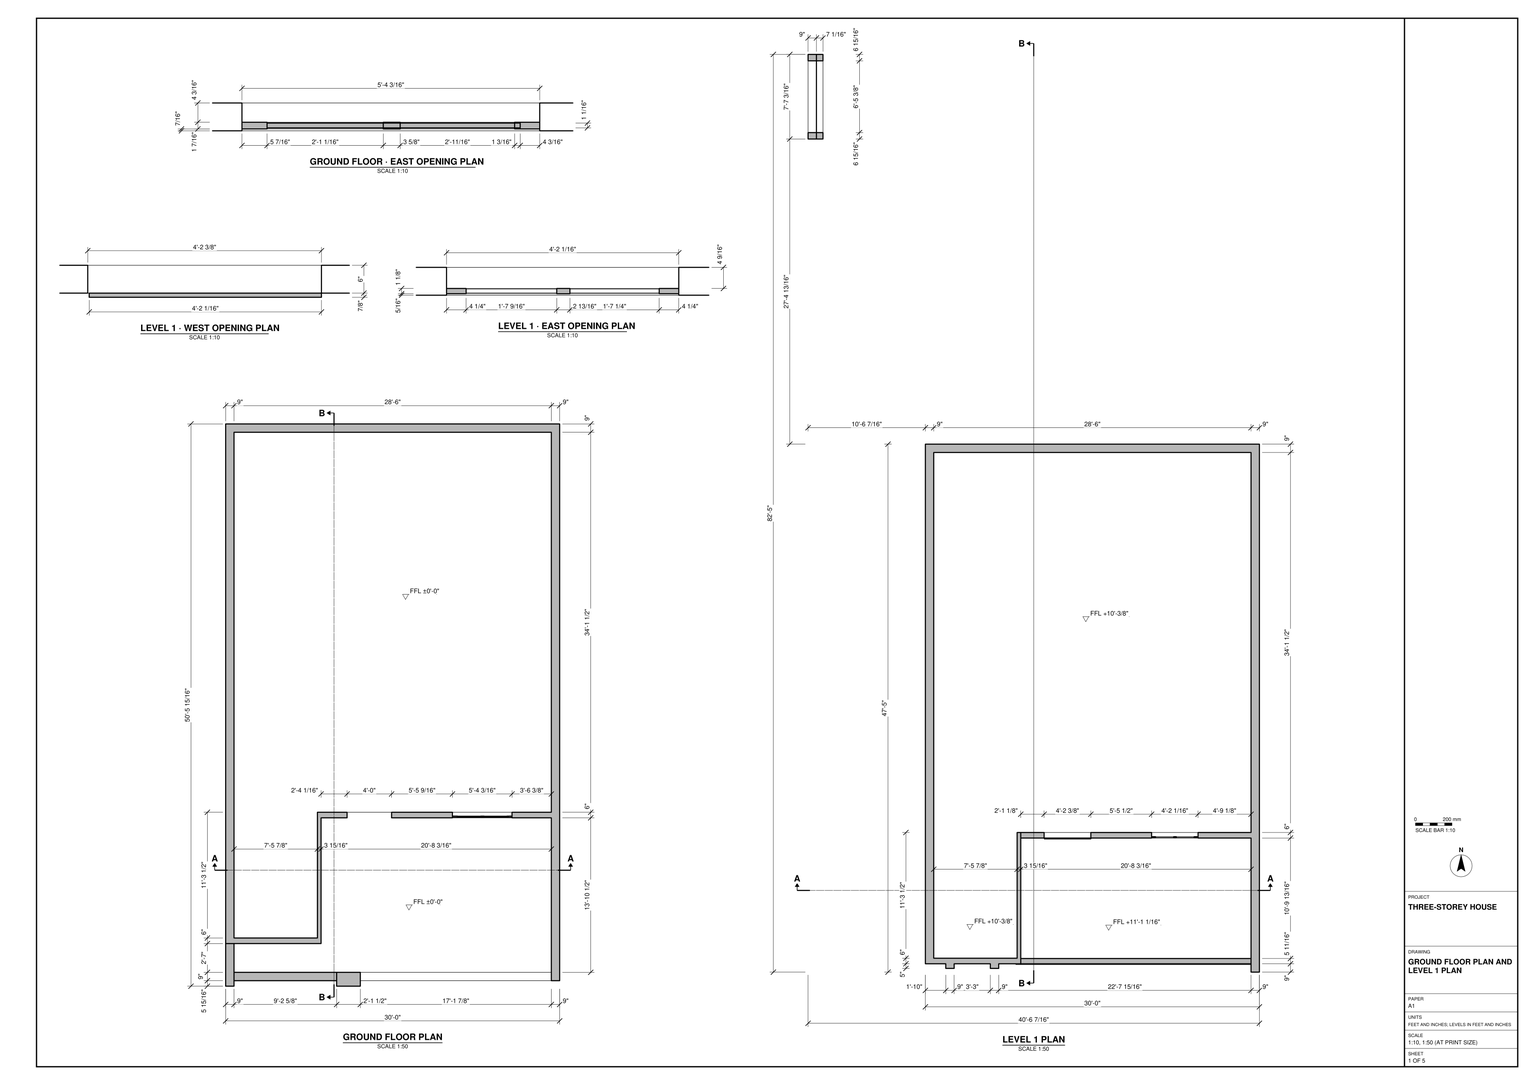
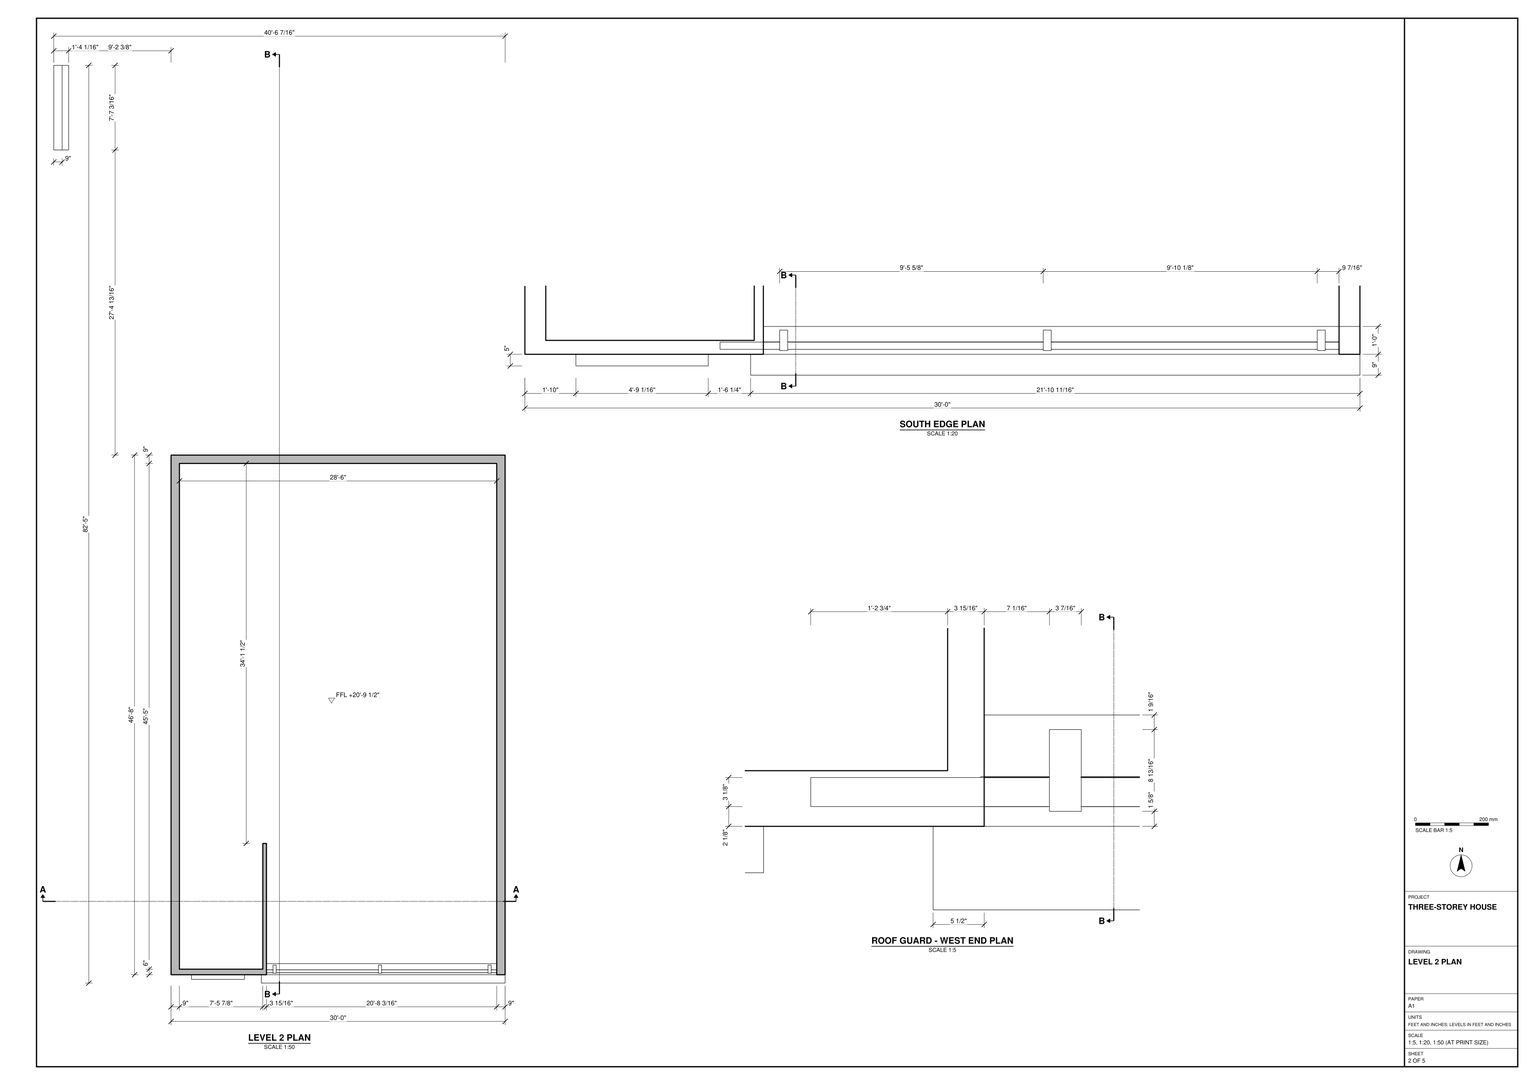
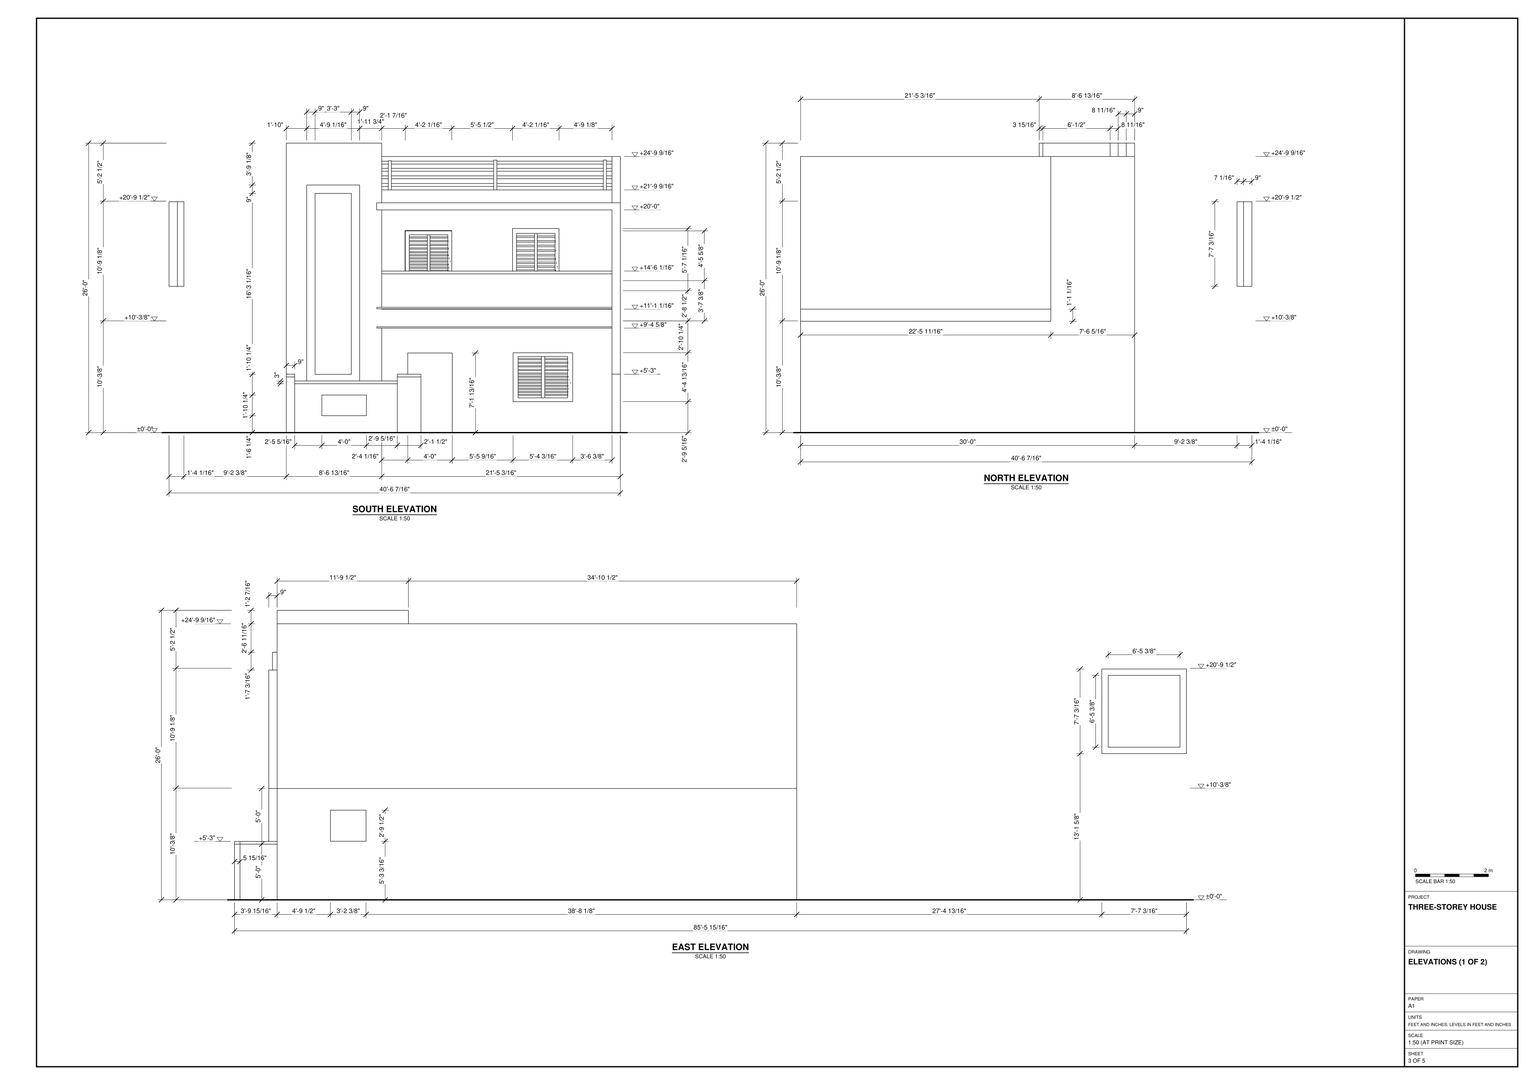
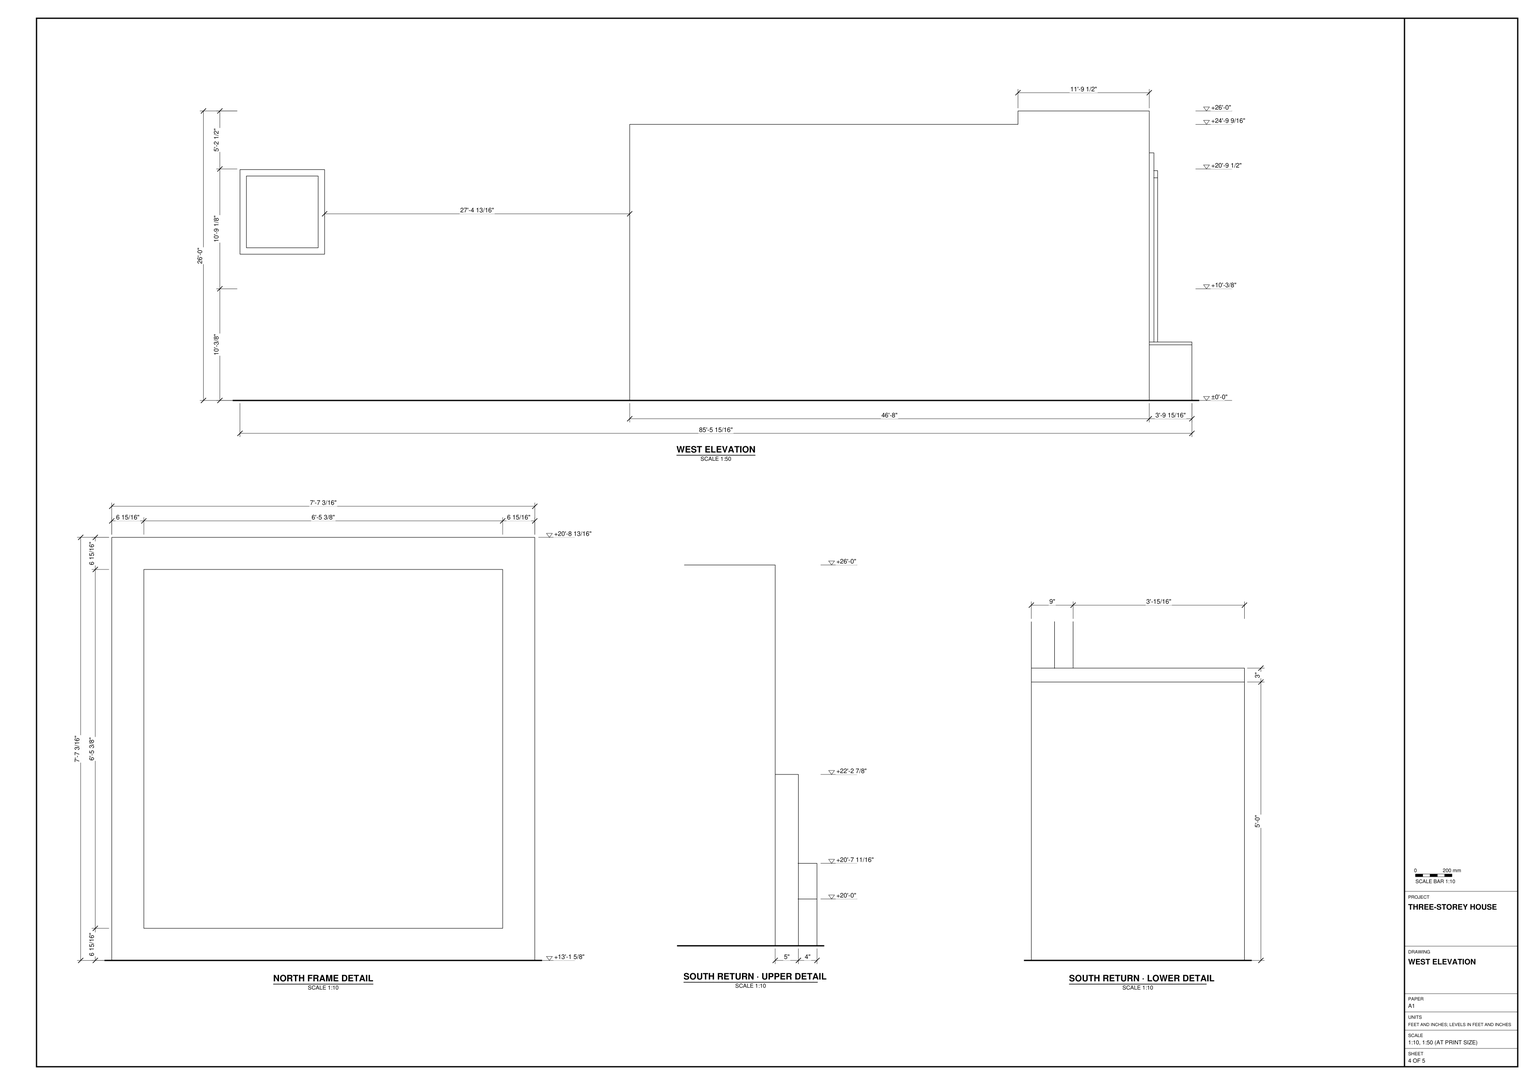
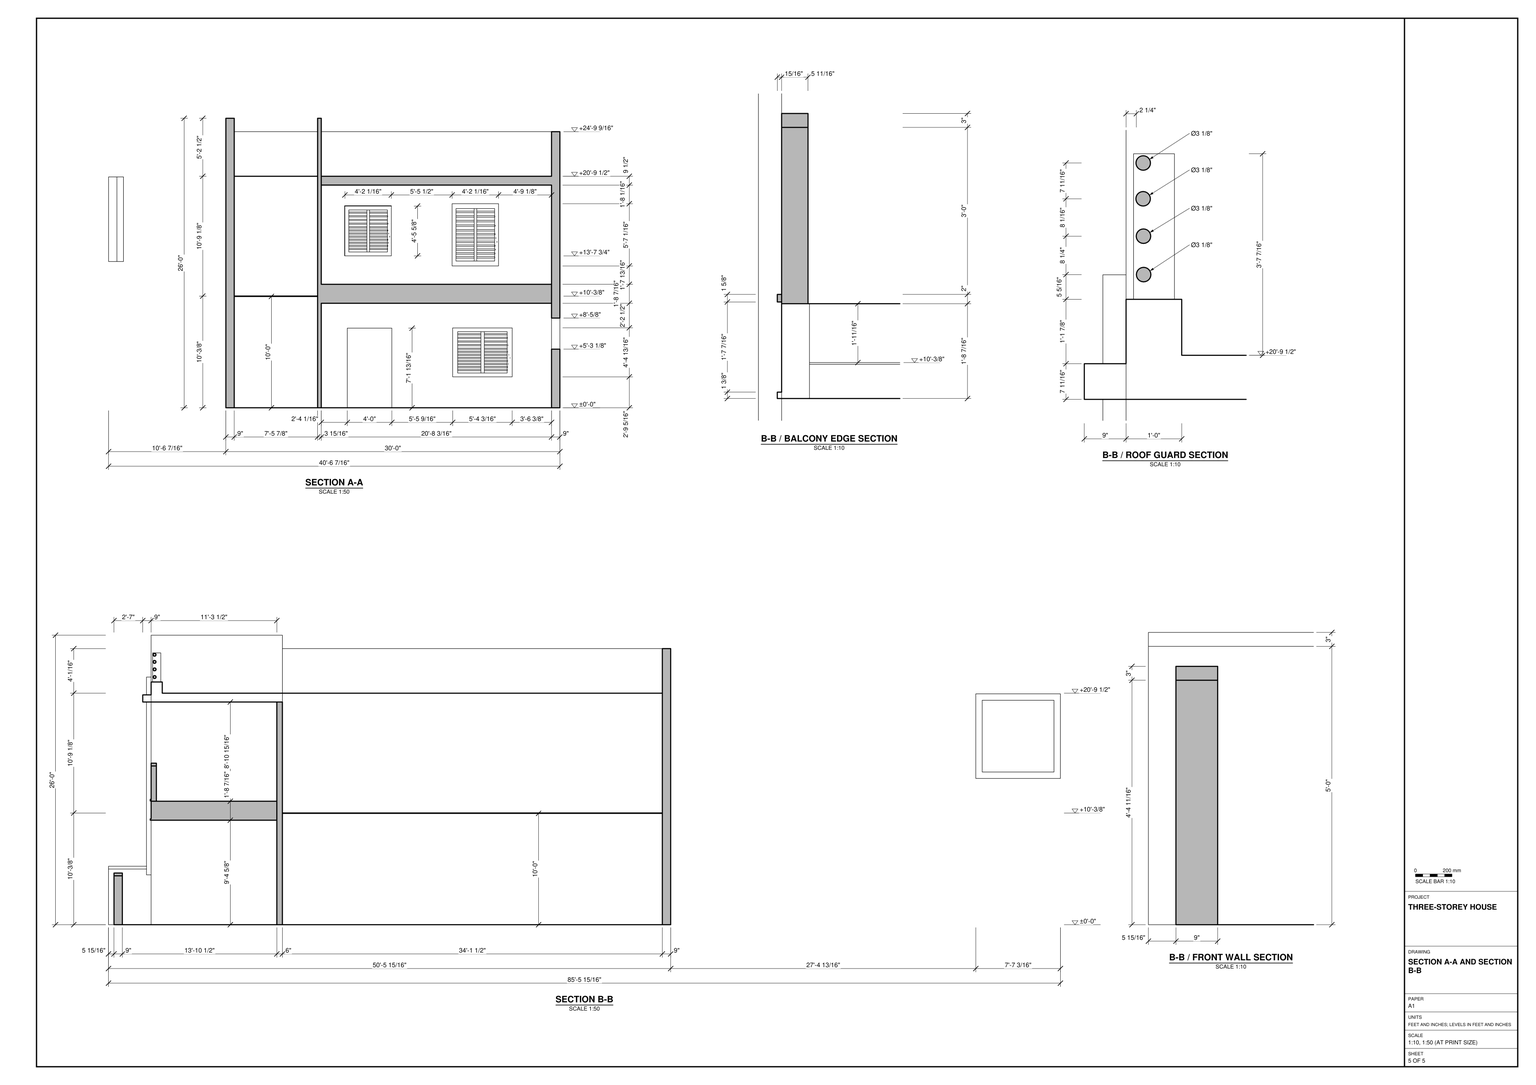
Build the three-storey house in SketchUp from task_files/diagram_01.pdf. Work in feet and inches. The overall model extents, including the detached rectangular frame northwest of the house, are 40'-6 7/16" east–west, 85'-5 15/16" north–south and 26'-0" high. Set the ground floor at ±0'-0", Level 1 at +10'-3/8" and Level 2 at +20'-9 1/2".

Lay out the long rectangular shell with the 9" perimeter walls and thinner wall returns shown in plan. Keep the large northern floor area open. At the south end, distinguish the narrow western bay from the wider recessed frontage. Model the ground-floor doorway and window, the low entrance wall and the tall framed panel on the western bay. Use the opening details to place the frames and divisions. At Level 1, show the change in slab level, the balcony front and the openings behind it. Form the flat roof terrace with its solid perimeter walls and the horizontal guard rails across the open part of the south edge. Use the elevations to position the detached frame above ground.

Keep walls, slabs and roof elements in separate groups or components; treat each furniture or joinery piece shown likewise and use components for repeated parts. Any decor or loose items shown may use suitable library components. Save one SketchUp model as output_files/three_storey_house_with_a_roof_terrace.skp.

# SketchUp Ruby script. Lengths in inches.
U = 1.inch
M = Sketchup.active_model
def pt(a) = Geom::Point3d.new(a.map { |v| v * U })
def face(e, loops, mat)
  f = e.add_face(loops[0].map { |a| pt(a) })
  loops[1..].each { |l| e.add_face(l.map { |a| pt(a) }).erase! }
  f.material = f.back_material = mat if mat
  f
end
# faces: each face lists its corners as indices into pts; further lists are holes
def faces(e, pts, list, mat = nil) = list.each { |f| face(e, (f[0].is_a?(Array) ? f : [f]).map { |l| l.map { |i| pts[i] } }, mat) }
# xy, xz, yz: faces in a plane at the given z, y or x. An outline is a flat list of corners, or four numbers for a rectangle; further outlines are holes
def ring(l) = l.size == 4 ? [[l[0], l[1]], [l[2], l[1]], [l[2], l[3]], [l[0], l[3]]] : l.each_slice(2).to_a
def flat(e, list, mat, &to3) = list.each { |f| face(e, (f[0].is_a?(Array) ? f : [f]).map { |l| ring(l).map { |u, v| to3.(u, v) } }, mat) }
def xy(e, z, list, mat = nil) = flat(e, list, mat) { |x, y| [x, y, z] }
def xz(e, y, list, mat = nil) = flat(e, list, mat) { |x, z| [x, y, z] }
def yz(e, x, list, mat = nil) = flat(e, list, mat) { |y, z| [x, y, z] }
def lines(e, pts, list) = list.each { |a, b| e.add_line(pt(pts[a]), pt(pts[b])) }
# prism: a flat outline (further loops are holes) pulled along v
def prism(e, loops, v, mat = nil)
  f = face(e, loops, mat); d = Geom::Vector3d.new(v.map { |x| x * U })
  f.pushpull(f.normal.samedirection?(d) ? d.length : -d.length)
end
def box(e, o, s, mat = nil) = prism(e, [[o, [o[0] + s[0], o[1], o[2]], [o[0] + s[0], o[1] + s[1], o[2]], [o[0], o[1] + s[1], o[2]]]], [0, 0, s[2]], mat)
def at(x, y, z, deg = 0) = Geom::Transformation.translation(pt([x, y, z])) * Geom::Transformation.rotation(ORIGIN, Z_AXIS, deg.degrees)
def axes(o, x, y, z) = Geom::Transformation.new([*x, 0, *y, 0, *z, 0, *pt(o).to_a, 1])
def part(name) = M.definitions.add(name)
# library, detail: a bought-in or finely detailed component or shape, given as its bounding box
def library(name, o, s) = part(name).tap { |d| box(d.entities, o, s) }
def detail(e, o, s) = box(e.add_group.entities, o, s)
def put(e, d, t, mat = nil) = e.add_instance(d, t).tap { |i| i.material = mat if mat }
def group(e, t, mat = nil) = e.add_group.tap { |g| g.transformation = t; g.material = mat if mat }.entities
root = M.entities
M.materials.add("[Color C08]").color = [102, 51, 0]
M.materials.add("[Color M05]").color = [114, 114, 114]
M.materials.add("[Translucent Glass Gray]").color = [128, 128, 128]
M.materials["[Translucent Glass Gray]"].alpha = 0.5
c1 = library("Group\#1",[0,0,0],[165.5,6.0625,179.125])
xy(root,0,[[126.43,0,135.43,45.9375],[246.05,0,271.56,14.9375],[135.43,5.9375,246.05,14.9375],[271.56,5.9375,477.43,14.9375],[477.43,5.9375,486.43,45.9375],
  [135.43,14.9375,477.43,14.9375,477.43,181.4375,305.29,181.4375,305.29,187.4375,257.29,187.4375,257.29,181.4375,229.25,181.4375,229.25,45.9375,135.43,45.9375],[126.43,45.9375,126.43,605.9375,486.43,605.9375,486.43,45.9375,477.43,45.9375,477.43,181.4375,305.29,181.4375,305.29,187.4375,477.43,187.4375,477.43,596.9375,135.43,596.9375,135.43,51.9375,225.31,51.9375,225.31,187.4375,257.29,187.4375,257.29,181.4375,229.25,181.4375,229.25,45.9375],[135.43,51.9375,225.31,51.9375,225.31,187.4375,477.43,187.4375,477.43,596.9375,135.43,596.9375]])
xy(root,18.26,[[164.74,5.9375,212.74,9.125]],"[Color M05]")
xy(root,33.34,[[370.86,181.4375,435.05,187.4375]])
xy(root,40.51,[[164.74,5.9375,212.74,9.125]],"[Color M05]")
xy(root,52.6875,[[135.43,5.9375,246.05,14.9375]])
xy(root,53.73,[[148.41,40.9375,205.47,45.9375]],"[Color C08]")
xy(root,55.6875,[[135.43,5.9375,246.05,14.9375]],"[Color M05]")
xy(root,60,[[126.43,0,135.43,45.9375],[246.05,0,271.56,14.9375]])
xy(root,62.75,[[157.43,40.9375,196.45,45.9375]],"[Color C08]")
xy(root,63,[[477.43,5.9375,486.43,36.9375]])
xy(root,63,[[126.43,0,135.43,45.9375],[246.05,0,271.56,14.9375]],"[Color M05]")
xy(root,63.17,[[477.43,103.41,486.43,141.79]])
xy(root,85.8125,[[257.29,181.4375,305.29,187.4375]])
xy(root,86.03,[[370.86,181.4375,435.05,187.4375]])
xy(root,96.67,[[477.43,103.41,486.43,141.79]])
xy(root,112.625,[[224,45,224,45.9375,229.25,45.9375,229.25,181.4375,477.43,181.4375,477.43,45]],"[Color C08]")
xy(root,114,[[224,45,477.43,45.9375]],"[Color C08]")
xy(root,120,[[135.43,51.9375,135.43,596.9375,477.43,596.9375,477.43,187.4375,225.31,187.4375,225.31,51.9375]])
xy(root,120.375,[[135.43,51.9375,225.31,51.9375,225.31,187.4375,477.43,187.4375,477.43,596.9375,135.43,596.9375]])
xy(root,133.0625,[[229.25,45.9375,477.43,51.625],[229.25,51.625,477.43,181.4375]])
xy(root,133.4375,[[224,45,229.25,45.9375],[229.25,45,477.43,45.9375]])
xy(root,135.0625,[[224,45,477.43,45.9375]],"[Color C08]")
xy(root,152.87,[[370.26,181.4375,420.32,187.4375]])
xy(root,157.62,[[0,934.78,9,1025.96],[9,934.78,16.0625,1025.96]])
xy(root,163.73,[[254.39,181.4375,304.77,187.4375]])
xy(root,164.53,[[0,941.69,9,1019.05],[9,941.69,16.0625,1019.05]])
xy(root,171.0625,[[229.25,45.9375,477.43,51.625]])
xy(root,174.0625,[[229.25,45.9375,477.43,51.625]],"[Color C08]")
xy(root,217.79,[[254.39,181.4375,304.77,187.4375]])
xy(root,219.93,[[370.26,181.4375,420.32,187.4375]])
xy(root,240,[[229.25,45.9375,477.43,181.4375],[229.25,181.4375,477.43,187.4375]])
xy(root,240,[[223.75,36.9375,477.43,45.9375]],"[Color C08]")
xy(root,241.89,[[0,941.69,9,1019.05],[9,941.69,16.0625,1019.05]])
xy(root,247.6875,[[223.75,36.9375,486.43,45.9375]],"[Color C08]")
xy(root,248.81,[[0,934.78,9,1025.96],[9,934.78,16.0625,1025.96]])
xy(root,249.5,[[135.43,51.9375,225.31,51.9375,225.31,187.4375,229.25,187.4375,229.25,57.9375,477.43,57.9375,477.43,596.9375,135.43,596.9375]])
xy(root,257.83,[[157.43,40.9375,196.45,45.9375]],"[Color C08]")
xy(root,261.5625,[[[229.25,45.9375,477.43,57.9375],[236.28,47.56,239.72,56.37],[349.9,47.56,353.34,56.37],[468.03,47.56,471.47,56.37]]])
xy(root,266.85,[[148.41,40.9375,205.47,45.9375]],"[Color C08]")
xy(root,292.9375,[[236.28,47.56,239.72,56.37]])
xy(root,293.6875,[[349.9,47.56,353.34,56.37]])
xy(root,293.75,[[468.03,47.56,471.47,56.37]])
xy(root,297.5625,[[477.43,45.9375,486.43,45.9375,486.43,605.9375,126.43,605.9375,126.43,187.4375,135.43,187.4375,135.43,596.9375,477.43,596.9375]])
xy(root,312,[[126.43,45.9375,229.25,45.9375,229.25,187.4375,225.31,187.4375,225.31,51.9375,135.43,51.9375,135.43,187.4375,126.43,187.4375]])
xz(root,0,[[126.43,0,135.43,60],[246.05,0,271.56,60]])
xz(root,0,[[126.43,60,135.43,63],[246.05,60,271.56,63]],"[Color M05]")
xz(root,5.9375,[[[135.43,0,246.05,52.6875],[164.74,18.26,212.74,40.51]],[477.43,0,486.43,63]])
xz(root,5.9375,[[135.43,52.6875,246.05,55.6875]],"[Color M05]")
xz(root,9.125,[[164.74,18.26,212.74,40.51]],"[Color M05]")
xz(root,14.9375,[[135.43,0,246.05,52.6875],[246.05,0,271.56,60]])
xz(root,14.9375,[[135.43,52.6875,246.05,55.6875],[246.05,60,271.56,63]],"[Color M05]")
xz(root,36.9375,[[477.43,63,486.43,63,486.43,247.6875,223.75,247.6875,223.75,240,477.43,240]],"[Color C08]")
xz(root,40.9375,[[[148.41,53.73,205.47,266.85],[157.43,62.75,196.45,257.83]]],"[Color C08]")
xz(root,45,[[224,112.625,477.43,114],[224,133.4375,477.43,135.0625]],"[Color C08]")
xz(root,45.9375,[[126.43,0,135.43,60],[[135.43,0,229.25,0,229.25,112.625,224,112.625,224,114,477.43,114,477.43,133.0625,229.25,133.0625,229.25,133.4375,224,133.4375,224,135.0625,229.25,135.0625,229.25,240,223.75,240,223.75,247.6875,229.25,247.6875,229.25,312,126.43,312,126.43,63,135.43,63],[148.41,53.73,205.47,266.85]],[126.43,60,135.43,63],[157.43,62.75,196.45,257.83],[224,112.625,229.25,114],
  [229.25,133.0625,232.81,133.4375],[232.81,133.0625,235.31,133.4375],[235.31,133.0625,312.5,133.4375],[312.5,133.0625,315.79,133.4375],[315.79,133.0625,392.93,133.4375],
  [392.93,133.0625,394.81,133.4375],[394.81,133.0625,469.81,133.4375],[469.81,133.0625,472.37,133.4375],[472.37,133.0625,477.43,133.4375],[224,133.4375,229.25,135.0625],
  [229.25,133.4375,232.81,135.0625],[232.81,133.4375,235.31,135.0625],[235.31,133.4375,312.5,135.0625],[312.5,133.4375,315.79,135.0625],[315.79,133.4375,392.93,135.0625],
  [392.93,133.4375,394.81,135.0625],[394.81,133.4375,469.81,135.0625],[469.81,133.4375,472.37,135.0625],[472.37,133.4375,477.43,135.0625],[223.75,240,229.25,247.6875],
  [229.25,247.6875,477.43,261.5625],[477.43,247.6875,486.43,297.5625]])
xz(root,45.9375,[[229.25,171.0625,477.43,174.0625]],"[Color C08]")
xz(root,45.9375,[[229.25,135.0625,477.43,171.0625]],"[Translucent Glass Gray]")
xz(root,47.56,[[236.28,261.5625,239.72,292.9375],[349.9,261.5625,353.34,293.6875],[468.03,261.5625,471.47,293.75]])
xz(root,51.625,[[229.25,171.0625,477.43,174.0625]],"[Color C08]")
xz(root,51.625,[[229.25,133.0625,477.43,171.0625]],"[Translucent Glass Gray]")
xz(root,51.9375,[[135.43,0,225.31,120],[135.43,120,152.81,120.375],[152.81,120,225.31,120.375],[135.43,120.375,152.81,249.5],[152.81,120.375,225.31,249.5],
  [135.43,249.5,144.12,312],[144.12,249.5,152.81,312],[152.81,249.5,225.31,312]])
xz(root,56.37,[[236.28,261.5625,239.72,292.9375],[349.9,261.5625,353.34,293.6875],[468.03,261.5625,471.47,293.75]])
xz(root,57.9375,[[229.25,249.5,477.43,261.5625]])
xz(root,103.41,[[477.43,63.17,486.43,96.67]])
xz(root,141.79,[[477.43,63.17,486.43,96.67]])
xz(root,181.4375,[[[229.25,0,257.29,0,257.29,85.8125,305.29,85.8125,305.29,0,477.43,0,477.43,112.625,229.25,112.625],[370.86,33.34,435.05,86.03]],[229.25,112.625,477.43,120],[229.25,120,477.43,133.0625],[[229.25,133.0625,477.43,240],[370.26,152.87,420.32,219.93],[254.39,163.73,304.77,217.79]]])
xz(root,187.4375,[[[225.31,0,225.31,120,477.43,120,477.43,0,305.29,0,305.29,85.8125,257.29,85.8125,257.29,0],[370.86,33.34,435.05,86.03]],[225.31,120,229.25,120.375],[229.25,120,477.43,120.375],[225.31,120.375,229.25,249.5],[229.25,120.375,477.43,133.0625],
  [[229.25,133.0625,477.43,240],[370.26,152.87,420.32,219.93],[254.39,163.73,304.77,217.79]],[225.31,249.5,229.25,312],[126.43,297.5625,135.43,312]])
xz(root,596.9375,[[135.43,0,477.43,120],[135.43,120,216.75,120.375],[216.75,120,477.43,120.375],[135.43,120.375,477.43,249.5],[135.43,249.5,477.43,297.5625]])
xz(root,605.9375,[[126.43,0,126.43,297.5625,216.75,297.5625,216.75,120,486.43,120,486.43,0],[216.75,120,486.43,133.0625],[216.75,133.0625,486.43,297.5625]])
xz(root,934.78,[[0,157.62,9,248.81],[9,157.62,16.0625,248.81]])
xz(root,941.69,[[0,164.53,9,241.89],[9,164.53,16.0625,241.89]])
xz(root,1019.05,[[0,164.53,9,241.89],[9,164.53,16.0625,241.89]])
xz(root,1025.96,[[0,157.62,9,248.81],[9,157.62,16.0625,248.81]])
yz(root,0,[[[934.78,157.62,1025.96,248.81],[941.69,164.53,1019.05,241.89]]])
yz(root,9,[[[934.78,157.62,1025.96,248.81],[941.69,164.53,1019.05,241.89]],[941.69,164.53,1019.05,241.89]])
yz(root,16.0625,[[[934.78,157.62,1025.96,248.81],[941.69,164.53,1019.05,241.89]]])
yz(root,126.43,[[0,0,45.9375,60],[45.9375,0,45.9375,312,187.4375,312,187.4375,297.5625,605.9375,297.5625,605.9375,0]])
yz(root,126.43,[[0,60,45.9375,63]],"[Color M05]")
yz(root,135.43,[[0,0,5.9375,0,5.9375,55.6875,14.9375,55.6875,14.9375,0,45.9375,0,45.9375,60,0,60],[5.9375,0,14.9375,52.6875],[51.9375,0,596.9375,120],[5.9375,52.6875,14.9375,55.6875],[51.9375,120,596.9375,120.375],
  [51.9375,120.375,596.9375,249.5],[51.9375,249.5,596.9375,249.5,596.9375,297.5625,187.4375,297.5625,187.4375,312,51.9375,312]])
yz(root,135.43,[[0,60,45.9375,63]],"[Color M05]")
yz(root,148.41,[[40.9375,53.73,45.9375,266.85]],"[Color C08]")
yz(root,157.43,[[40.9375,62.75,45.9375,257.83]],"[Color C08]")
yz(root,164.74,[[5.9375,18.26,9.125,40.51]],"[Color M05]")
yz(root,196.45,[[40.9375,62.75,45.9375,257.83]],"[Color C08]")
yz(root,205.47,[[40.9375,53.73,45.9375,266.85]],"[Color C08]")
yz(root,210.56,[[49.63,289.39,49.23,289.44,48.85,289.6,48.53,289.85,48.28,290.17,48.125,290.55,48.07,290.95,48.125,291.36,48.28,291.73,48.53,292.06,48.85,292.3,49.23,292.46,49.63,292.51,50.04,292.46,50.42,292.3,50.74,292.06,50.99,291.73,51.14,291.36,51.2,290.95,51.14,290.55,50.99,290.17,50.74,289.85,50.42,289.6,50.04,289.44]])
yz(root,212.74,[[5.9375,18.26,9.125,40.51]],"[Color M05]")
yz(root,223.75,[[36.9375,240,45.9375,247.6875]],"[Color C08]")
yz(root,224,[[45,112.625,45.9375,114],[45,133.4375,45.9375,135.0625]],"[Color C08]")
yz(root,225.31,[[51.9375,0,187.4375,120],[51.9375,120,187.4375,120.375],[51.9375,120.375,187.4375,249.5],[51.9375,249.5,187.4375,312]])
yz(root,228.87,[[49.73,265.33,49.32,265.39,48.94,265.54,48.62,265.79,48.37,266.12,48.22,266.49,48.16,266.9,48.22,267.3,48.37,267.68,48.62,268,48.94,268.25,49.32,268.41,49.73,268.46,50.13,268.41,50.51,268.25,50.83,268,51.08,267.68,51.24,267.3,51.29,266.9,51.24,266.49,51.08,266.12,50.83,265.79,50.51,265.54,50.13,265.39]])
yz(root,229.25,[[45.9375,0,181.4375,112.625],[181.4375,120,187.4375,133.0625],[45.9375,133.0625,51.625,171.0625],[51.625,133.0625,181.4375,133.0625,181.4375,240,45.9375,240,45.9375,174.0625,51.625,174.0625],[181.4375,133.0625,187.4375,240],
  [45.9375,171.0625,51.625,174.0625],[45.9375,240,187.4375,240,187.4375,249.5,57.9375,249.5,57.9375,261.5625,45.9375,261.5625],[[57.9375,249.5,187.4375,249.5,187.4375,312,45.9375,312,45.9375,261.5625,57.9375,261.5625],[49.69,273.61,49.29,273.66,48.91,273.82,48.59,274.07,48.34,274.39,48.18,274.77,48.13,275.17,48.18,275.58,48.34,275.96,48.59,276.28,48.91,276.53,49.29,276.68,49.69,276.74,50.1,276.68,50.47,276.53,50.8,276.28,51.04,275.96,51.2,275.58,51.25,275.17,51.2,274.77,51.04,274.39,50.8,274.07,50.47,273.82,50.1,273.66],[49.62,281.68,49.21,281.73,48.84,281.89,48.51,282.13,48.26,282.46,48.11,282.83,48.05,283.24,48.11,283.64,48.26,284.02,48.51,284.34,48.84,284.59,49.21,284.75,49.62,284.8,50.02,284.75,50.4,284.59,50.72,284.34,50.97,284.02,51.125,283.64,51.18,283.24,51.125,282.83,50.97,282.46,50.72,282.13,50.4,281.89,50.02,281.73]]])
yz(root,236.28,[[47.56,261.5625,56.37,292.9375]])
yz(root,239.72,[[47.56,261.5625,56.37,292.9375]])
yz(root,246.05,[[0,0,0,60,14.9375,60,14.9375,55.6875,5.9375,55.6875,5.9375,0],[5.9375,0,14.9375,52.6875],[5.9375,52.6875,14.9375,55.6875]])
yz(root,246.05,[[0,60,14.9375,63]],"[Color M05]")
yz(root,254.39,[[181.4375,163.73,187.4375,217.79]])
yz(root,257.29,[[181.4375,0,187.4375,85.8125]])
yz(root,271.56,[[0,0,14.9375,60]])
yz(root,271.56,[[0,60,14.9375,63]],"[Color M05]")
yz(root,304.77,[[181.4375,163.73,187.4375,217.79]])
yz(root,305.29,[[181.4375,0,187.4375,85.8125]])
yz(root,349.9,[[47.56,261.5625,56.37,293.6875]])
yz(root,353.34,[[47.56,261.5625,56.37,293.6875]])
yz(root,370.26,[[181.4375,152.87,187.4375,219.93]])
yz(root,370.86,[[181.4375,33.34,187.4375,86.03]])
yz(root,420.32,[[181.4375,152.87,187.4375,219.93]])
yz(root,435.05,[[181.4375,33.34,187.4375,86.03]])
yz(root,468.03,[[47.56,261.5625,56.37,293.75]])
yz(root,471.47,[[47.56,261.5625,56.37,293.75]])
yz(root,477.43,[[[5.9375,0,5.9375,63,36.9375,63,36.9375,240,181.4375,240,181.4375,133.0625,51.625,133.0625,51.625,174.0625,45.9375,174.0625,45.9375,135.0625,45,135.0625,45,133.4375,45.9375,133.4375,45.9375,114,45,114,45,112.625,181.4375,112.625,181.4375,0],[103.41,63.17,141.79,96.67]],[187.4375,0,596.9375,120],[45,112.625,45.9375,114],[45.9375,112.625,181.4375,120],[45.9375,120,181.4375,133.0625],
  [187.4375,120,596.9375,120.375],[187.4375,120.375,596.9375,249.5],[45.9375,133.0625,51.625,171.0625],[45,133.4375,45.9375,135.0625],[45.9375,171.0625,51.625,174.0625],
  [57.9375,249.5,596.9375,297.5625],[[45.9375,261.5625,57.9375,297.5625],[49.73,265.33,50.13,265.39,50.51,265.54,50.83,265.79,51.08,266.12,51.24,266.49,51.29,266.9,51.24,267.3,51.08,267.68,50.83,268,50.51,268.25,50.13,268.41,49.73,268.46,49.32,268.41,48.94,268.25,48.62,268,48.37,267.68,48.22,267.3,48.16,266.9,48.22,266.49,48.37,266.12,48.62,265.79,48.94,265.54,49.32,265.39],[49.69,273.61,50.1,273.66,50.47,273.82,50.8,274.07,51.04,274.39,51.2,274.77,51.25,275.17,51.2,275.58,51.04,275.96,50.8,276.28,50.47,276.53,50.1,276.68,49.69,276.74,49.29,276.68,48.91,276.53,48.59,276.28,48.34,275.96,48.18,275.58,48.13,275.17,48.18,274.77,48.34,274.39,48.59,274.07,48.91,273.82,49.29,273.66],[49.62,281.68,50.02,281.73,50.4,281.89,50.72,282.13,50.97,282.46,51.125,282.83,51.18,283.24,51.125,283.64,50.97,284.02,50.72,284.34,50.4,284.59,50.02,284.75,49.62,284.8,49.21,284.75,48.84,284.59,48.51,284.34,48.26,284.02,48.11,283.64,48.05,283.24,48.11,282.83,48.26,282.46,48.51,282.13,48.84,281.89,49.21,281.73],[49.63,289.39,50.04,289.44,50.42,289.6,50.74,289.85,50.99,290.17,51.14,290.55,51.2,290.95,51.14,291.36,50.99,291.73,50.74,292.06,50.42,292.3,50.04,292.46,49.63,292.51,49.23,292.46,48.85,292.3,48.53,292.06,48.28,291.73,48.125,291.36,48.07,290.95,48.125,290.55,48.28,290.17,48.53,289.85,48.85,289.6,49.23,289.44]],[49.73,265.33,50.13,265.39,50.51,265.54,50.83,265.79,51.08,266.12,51.24,266.49,51.29,266.9,51.24,267.3,51.08,267.68,50.83,268,50.51,268.25,50.13,268.41,49.73,268.46,49.32,268.41,48.94,268.25,48.62,268,48.37,267.68,48.22,267.3,48.16,266.9,48.22,266.49,48.37,266.12,48.62,265.79,48.94,265.54,49.32,265.39],[49.69,273.61,50.1,273.66,50.47,273.82,50.8,274.07,51.04,274.39,51.2,274.77,51.25,275.17,51.2,275.58,51.04,275.96,50.8,276.28,50.47,276.53,50.1,276.68,49.69,276.74,49.29,276.68,48.91,276.53,48.59,276.28,48.34,275.96,48.18,275.58,48.13,275.17,48.18,274.77,48.34,274.39,48.59,274.07,48.91,273.82,49.29,273.66],[49.62,281.68,50.02,281.73,50.4,281.89,50.72,282.13,50.97,282.46,51.125,282.83,51.18,283.24,51.125,283.64,50.97,284.02,50.72,284.34,50.4,284.59,50.02,284.75,49.62,284.8,49.21,284.75,48.84,284.59,48.51,284.34,48.26,284.02,48.11,283.64,48.05,283.24,48.11,282.83,48.26,282.46,48.51,282.13,48.84,281.89,49.21,281.73],
  [49.63,289.39,50.04,289.44,50.42,289.6,50.74,289.85,50.99,290.17,51.14,290.55,51.2,290.95,51.14,291.36,50.99,291.73,50.74,292.06,50.42,292.3,50.04,292.46,49.63,292.51,49.23,292.46,48.85,292.3,48.53,292.06,48.28,291.73,48.125,291.36,48.07,290.95,48.125,290.55,48.28,290.17,48.53,289.85,48.85,289.6,49.23,289.44]])
yz(root,486.43,[[5.9375,0,45.9375,60],[[45.9375,0,605.9375,120],[103.41,63.17,141.79,96.67]],[5.9375,60,45.9375,63],[36.9375,63,45.9375,120],[36.9375,120,45.9375,247.6875],
  [45.9375,120,605.9375,297.5625]])
p = [[477.43,49.73,265.33],[477.43,49.32,265.39],[228.87,49.32,265.39],[228.87,49.73,265.33],[477.43,50.13,265.39],[228.87,50.13,265.39],
  [477.43,48.94,265.54],[228.87,48.94,265.54],[477.43,50.51,265.54],[228.87,50.51,265.54],[477.43,48.62,265.79],[228.87,48.62,265.79],
  [477.43,50.83,265.79],[228.87,50.83,265.79],[477.43,48.37,266.12],[228.87,48.37,266.12],[477.43,51.08,266.12],[228.87,51.08,266.12],
  [477.43,48.22,266.49],[228.87,48.22,266.49],[477.43,51.24,266.49],[228.87,51.24,266.49],[477.43,48.16,266.9],[228.87,48.16,266.9],
  [477.43,51.29,266.9],[228.87,51.29,266.9],[477.43,48.22,267.3],[228.87,48.22,267.3],[477.43,51.24,267.3],[228.87,51.24,267.3],
  [477.43,48.37,267.68],[228.87,48.37,267.68],[477.43,51.08,267.68],[228.87,51.08,267.68],[477.43,48.62,268],[228.87,48.62,268],
  [477.43,50.83,268],[228.87,50.83,268],[477.43,48.94,268.25],[228.87,48.94,268.25],[477.43,50.51,268.25],[228.87,50.51,268.25],
  [477.43,49.32,268.41],[228.87,49.32,268.41],[477.43,50.13,268.41],[228.87,50.13,268.41],[477.43,49.73,268.46],[228.87,49.73,268.46],
  [477.43,49.69,273.61],[477.43,49.29,273.66],[229.25,49.29,273.66],[229.25,49.69,273.61],[477.43,50.1,273.66],[229.25,50.1,273.66],
  [477.43,48.91,273.82],[229.25,48.91,273.82],[477.43,50.47,273.82],[229.25,50.47,273.82],[477.43,48.59,274.07],[229.25,48.59,274.07],
  [477.43,50.8,274.07],[229.25,50.8,274.07],[477.43,48.34,274.39],[229.25,48.34,274.39],[477.43,51.04,274.39],[229.25,51.04,274.39],
  [477.43,48.18,274.77],[229.25,48.18,274.77],[477.43,51.2,274.77],[229.25,51.2,274.77],[477.43,48.13,275.17],[229.25,48.13,275.17],
  [477.43,51.25,275.17],[229.25,51.25,275.17],[477.43,48.18,275.58],[229.25,48.18,275.58],[477.43,51.2,275.58],[229.25,51.2,275.58],
  [477.43,48.34,275.96],[229.25,48.34,275.96],[477.43,51.04,275.96],[229.25,51.04,275.96],[477.43,48.59,276.28],[229.25,48.59,276.28],
  [477.43,50.8,276.28],[229.25,50.8,276.28],[477.43,48.91,276.53],[229.25,48.91,276.53],[477.43,50.47,276.53],[229.25,50.47,276.53],
  [477.43,49.29,276.68],[229.25,49.29,276.68],[477.43,50.1,276.68],[229.25,50.1,276.68],[477.43,49.69,276.74],[229.25,49.69,276.74],
  [477.43,49.21,281.73],[477.43,48.84,281.89],[229.25,48.84,281.89],[229.25,49.21,281.73],[477.43,49.62,281.68],[229.25,49.62,281.68],
  [477.43,50.02,281.73],[229.25,50.02,281.73],[477.43,50.4,281.89],[229.25,50.4,281.89],[477.43,48.51,282.13],[229.25,48.51,282.13],
  [477.43,50.72,282.13],[229.25,50.72,282.13],[477.43,48.26,282.46],[229.25,48.26,282.46],[477.43,50.97,282.46],[229.25,50.97,282.46],
  [477.43,48.11,282.83],[229.25,48.11,282.83],[477.43,51.125,282.83],[229.25,51.125,282.83],[477.43,48.05,283.24],[229.25,48.05,283.24],
  [477.43,51.18,283.24],[229.25,51.18,283.24],[477.43,48.11,283.64],[229.25,48.11,283.64],[477.43,51.125,283.64],[229.25,51.125,283.64],
  [477.43,48.26,284.02],[229.25,48.26,284.02],[477.43,50.97,284.02],[229.25,50.97,284.02],[477.43,48.51,284.34],[229.25,48.51,284.34],
  [477.43,50.72,284.34],[229.25,50.72,284.34],[477.43,48.84,284.59],[229.25,48.84,284.59],[477.43,50.4,284.59],[229.25,50.4,284.59],
  [477.43,49.21,284.75],[229.25,49.21,284.75],[477.43,50.02,284.75],[229.25,50.02,284.75],[477.43,49.62,284.8],[229.25,49.62,284.8],
  [477.43,49.23,289.44],[477.43,48.85,289.6],[210.56,48.85,289.6],[210.56,49.23,289.44],[477.43,49.63,289.39],[210.56,49.63,289.39],
  [477.43,50.04,289.44],[210.56,50.04,289.44],[477.43,50.42,289.6],[210.56,50.42,289.6],[477.43,48.53,289.85],[210.56,48.53,289.85],
  [477.43,50.74,289.85],[210.56,50.74,289.85],[477.43,48.28,290.17],[210.56,48.28,290.17],[477.43,50.99,290.17],[210.56,50.99,290.17],
  [477.43,48.125,290.55],[210.56,48.125,290.55],[477.43,51.14,290.55],[210.56,51.14,290.55],[477.43,48.07,290.95],[210.56,48.07,290.95],
  [477.43,51.2,290.95],[210.56,51.2,290.95],[477.43,48.125,291.36],[210.56,48.125,291.36],[477.43,51.14,291.36],[210.56,51.14,291.36],
  [477.43,48.28,291.73],[210.56,48.28,291.73],[477.43,50.99,291.73],[210.56,50.99,291.73],[477.43,48.53,292.06],[210.56,48.53,292.06],
  [477.43,50.74,292.06],[210.56,50.74,292.06],[477.43,48.85,292.3],[210.56,48.85,292.3],[477.43,50.42,292.3],[210.56,50.42,292.3],
  [477.43,49.23,292.46],[210.56,49.23,292.46],[477.43,50.04,292.46],[210.56,50.04,292.46],[477.43,49.63,292.51],[210.56,49.63,292.51],
  [477.43,45.9375,60],[486.43,45.9375,60],[477.43,45.9375,63],[486.43,45.9375,63],[216.75,596.9375,120],[216.75,605.9375,120],
  [216.75,596.9375,133.0625],[216.75,605.9375,133.0625],[477.43,57.9375,261.5625],[486.31,57.9375,261.5625]]
faces(root,p,[[0,1,2,3],[4,0,3,5],[1,6,7,2],[8,4,5,9],[6,10,11,7],[12,8,9,13],[10,14,15,11],[16,12,13,17],
  [14,18,19,15],[20,16,17,21],[18,22,23,19],[24,20,21,25],[22,26,27,23],[28,24,25,29],[26,30,31,27],[32,28,29,33],
  [30,34,35,31],[36,32,33,37],[34,38,39,35],[40,36,37,41],[38,42,43,39],[44,40,41,45],[42,46,47,43],[46,44,45,47],
  [48,49,50,51],[52,48,51,53],[49,54,55,50],[56,52,53,57],[54,58,59,55],[60,56,57,61],[58,62,63,59],[64,60,61,65],
  [62,66,67,63],[68,64,65,69],[66,70,71,67],[72,68,69,73],[70,74,75,71],[76,72,73,77],[74,78,79,75],[80,76,77,81],
  [78,82,83,79],[84,80,81,85],[82,86,87,83],[88,84,85,89],[86,90,91,87],[92,88,89,93],[90,94,95,91],[94,92,93,95],
  [96,97,98,99],[100,96,99,101],[102,100,101,103],[104,102,103,105],[97,106,107,98],[108,104,105,109],[106,110,111,107],[112,108,109,113],
  [110,114,115,111],[116,112,113,117],[114,118,119,115],[120,116,117,121],[118,122,123,119],[124,120,121,125],[122,126,127,123],[128,124,125,129],
  [126,130,131,127],[132,128,129,133],[130,134,135,131],[136,132,133,137],[134,138,139,135],[140,136,137,141],[138,142,143,139],[142,140,141,143],
  [144,145,146,147],[148,144,147,149],[150,148,149,151],[152,150,151,153],[145,154,155,146],[156,152,153,157],[154,158,159,155],[160,156,157,161],
  [158,162,163,159],[164,160,161,165],[162,166,167,163],[168,164,165,169],[166,170,171,167],[172,168,169,173],[170,174,175,171],[176,172,173,177],
  [174,178,179,175],[180,176,177,181],[178,182,183,179],[184,180,181,185],[182,186,187,183],[188,184,185,189],[186,190,191,187],[190,188,189,191]])
lines(root,p,[[192,193],[194,195],[196,197],[198,199],[200,201]])
put(root,c1,axes([370.86,181.83,33.34],[0.38784,0,0],[0,0.2397,0],[0,0,0.29484]))
put(root,c1,axes([370.26,181.76,152.87],[0.30252,0,0],[0,0.18697,0],[0,0,0.37439]))
put(root,c1,axes([254.7,180.53,163.73],[0.30252,0,0],[0,0.14958,0],[0,0,0.29951]))
